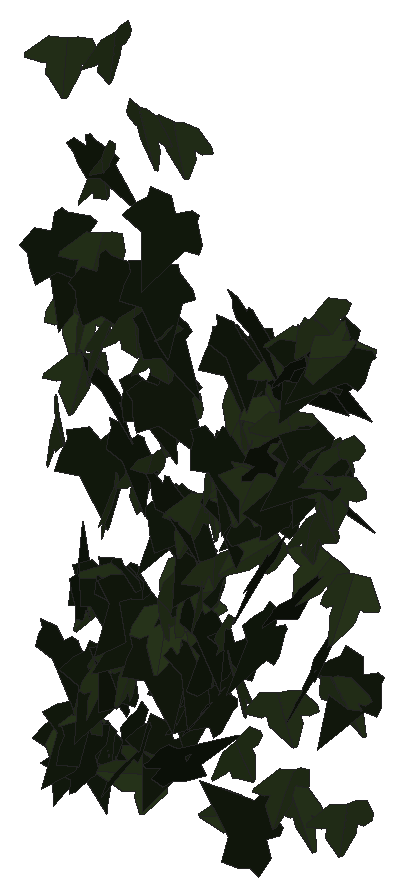
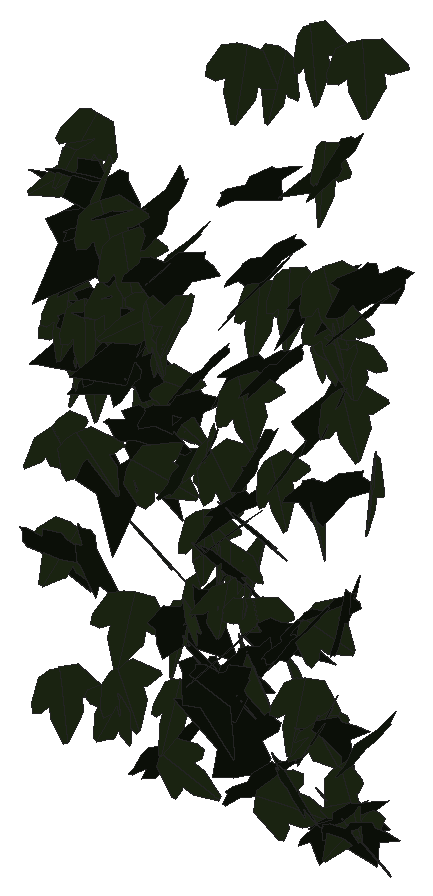
# SketchUp Ruby script. Lengths in inches.
U = 1.inch
M = Sketchup.active_model
def pt(a) = Geom::Point3d.new(a.map { |v| v * U })
def face(e, loops, mat)
  f = e.add_face(loops[0].map { |a| pt(a) })
  loops[1..].each { |l| e.add_face(l.map { |a| pt(a) }).erase! }
  f.material = f.back_material = mat if mat
  f
end
# faces: each face lists its corners as indices into pts; further lists are holes
def faces(e, pts, list, mat = nil) = list.each { |f| face(e, (f[0].is_a?(Array) ? f : [f]).map { |l| l.map { |i| pts[i] } }, mat) }
# xy, xz, yz: faces in a plane at the given z, y or x. An outline is a flat list of corners, or four numbers for a rectangle; further outlines are holes
def ring(l) = l.size == 4 ? [[l[0], l[1]], [l[2], l[1]], [l[2], l[3]], [l[0], l[3]]] : l.each_slice(2).to_a
def flat(e, list, mat, &to3) = list.each { |f| face(e, (f[0].is_a?(Array) ? f : [f]).map { |l| ring(l).map { |u, v| to3.(u, v) } }, mat) }
def xy(e, z, list, mat = nil) = flat(e, list, mat) { |x, y| [x, y, z] }
def xz(e, y, list, mat = nil) = flat(e, list, mat) { |x, z| [x, y, z] }
def yz(e, x, list, mat = nil) = flat(e, list, mat) { |y, z| [x, y, z] }
def lines(e, pts, list) = list.each { |a, b| e.add_line(pt(pts[a]), pt(pts[b])) }
# prism: a flat outline (further loops are holes) pulled along v
def prism(e, loops, v, mat = nil)
  f = face(e, loops, mat); d = Geom::Vector3d.new(v.map { |x| x * U })
  f.pushpull(f.normal.samedirection?(d) ? d.length : -d.length)
end
def box(e, o, s, mat = nil) = prism(e, [[o, [o[0] + s[0], o[1], o[2]], [o[0] + s[0], o[1] + s[1], o[2]], [o[0], o[1] + s[1], o[2]]]], [0, 0, s[2]], mat)
def at(x, y, z, deg = 0) = Geom::Transformation.translation(pt([x, y, z])) * Geom::Transformation.rotation(ORIGIN, Z_AXIS, deg.degrees)
def axes(o, x, y, z) = Geom::Transformation.new([*x, 0, *y, 0, *z, 0, *pt(o).to_a, 1])
def part(name) = M.definitions.add(name)
# library, detail: a bought-in or finely detailed component or shape, given as its bounding box
def library(name, o, s) = part(name).tap { |d| box(d.entities, o, s) }
def detail(e, o, s) = box(e.add_group.entities, o, s)
def put(e, d, t, mat = nil) = e.add_instance(d, t).tap { |i| i.material = mat if mat }
def group(e, t, mat = nil) = e.add_group.tap { |g| g.transformation = t; g.material = mat if mat }.entities
root = M.entities
M.materials.add("efeu1").color = [18, 25, 13]
M.materials.add("efeu2").color = [43, 57, 29]
c1 = part("ivyleaf_10")
p = [[0,0.5,-0.03],[-0.0625,2.02,-0.43],[-0.19,2.01,-0.46],[-0.54,1.05,-0.29],[-0.52,0.625,-0.18],[-0.83,0.76,-0.28],
  [-1.16,0.64,-0.33],[-1.15,0.33,-0.24],[-0.77,-0.39,0.02],[-0.3,-0.51,0.16],[0.04,-0.48,0.23],[-0.02,2.01,-0.4375],
  [-0.06,2.01,-0.43],[0.04,-0.49,0.23],[0.67,-0.49,0.14],[1.38,0.36,-0.2],[1.375,0.51,-0.24],[0.81,0.65,-0.19],
  [0.62,0.59,-0.15],[0.6,1.09,-0.28],[0.5,1.23,-0.31]]
faces(c1.entities,p,[[0,1,2,3,4,5,6,7,8,9,10],[11,12,0,13,14,15,16,17,18,19,20]],"efeu2")
c2 = part("ivyleaf_9")
p = [[1.54,2.16,1.25],[1.36,2.04,1.19],[-0.21,0.99,0.68],[-0.71,1.11,0.82],[-0.85,0.86,0.67],[-0.8,0.17,0.21],
  [-0.9,-0.01,0.1],[-0.67,-0.16,-0.02],[-0.08,-0.08,-0.05],[-0.03,-0.6,-0.4],[0.65,-0.88,-0.66],[0.83,-0.6,-0.49],
  [1.29,-0.42,-0.43],[1.8125,-0.07,-0.26],[1.21,0.44,0.15]]
faces(c2.entities,p,[[0,1,2,3,4,5,6,7,8,9,10,11,12,13,14]],"efeu1")
put(root,c1,axes([562.84,127.59,257.41],[0.41303,-0.76351,-0.7131],[-0.09509,0.73616,-0.84327],[1.0404,0.37039,0.20603]))
put(root,c2,axes([562.25,128.91,247.09],[0.18031,-0.95699,0.36294],[0.20425,-0.32748,-0.96494],[1.00292,0.23875,0.13126]))
put(root,c2,axes([562.58,127.88,265.38],[0.22614,-0.63801,-0.89851],[0.05984,0.92299,-0.64034],[1.10036,0.08093,0.21948]))
put(root,c2,axes([563.07,128.88,243.53],[-0.73357,-0.65535,-0.20186],[0.21145,0.06502,-0.9795],[0.65232,-0.75806,0.09049]))
put(root,c1,axes([563.75,128.37,244.99],[-0.7587,0.15917,0.7499],[-0.74689,0.08426,-0.77354],[-0.17274,-1.06342,0.05095]))
put(root,c2,axes([562.89,128.7,263.84],[-0.16436,-1.00943,0.40946],[0.11007,-0.42737,-1.00939],[1.08374,-0.10968,0.16461]))
put(root,c1,axes([563.41,127.64,273.79],[-0.83592,-0.75041,0.11104],[-0.01136,-0.15283,-1.11835],[0.75849,-0.8293,0.10562]))
put(root,c2,axes([563.48,129.04,243.86],[-0.63138,-0.80957,0.35535],[-0.14365,-0.33692,-1.02282],[0.87238,-0.6414,0.08876]))
put(root,c1,axes([563.04,128.13,243.67],[0.40834,0.68659,0.64921],[0.32372,0.56279,-0.79881],[-0.88774,0.52104,0.00733]))
put(root,c1,axes([563.73,128.17,259.99],[-0.44641,-0.98521,0.21774],[-0.00764,-0.2348,-1.07802],[1.00895,-0.43768,0.08817]))
put(root,c1,axes([563.39,128.36,262.37],[1.04935,0.34469,0.06041],[0.06179,0.00547,-1.10443],[-0.34445,1.05108,-0.01407]))
put(root,c1,axes([563.98,128.51,263.49],[-1.02158,-0.29347,0.28723],[-0.25696,-0.14386,-1.06091],[0.32031,-1.0514,0.06499]))
put(root,c2,axes([564.42,127.89,243.42],[-0.78664,0.6294,0.42305],[-0.35232,0.23647,-1.00692],[-0.67156,-0.86131,0.03271]))
put(root,c1,axes([564.05,128.8,265.03],[-0.49407,-0.95007,0.25956],[0.00953,-0.29498,-1.06161],[0.98484,-0.47378,0.14048]))
put(root,c2,axes([563.69,128.74,243.64],[0.0197,-0.96646,-0.33025],[0.01052,0.33048,-0.96652],[1.02127,0.01524,0.01633]))
put(root,c1,axes([564,128.18,263.08],[0.45011,-0.89395,0.51532],[0.33214,-0.40677,-0.99575],[0.97693,0.55017,0.10111]))
put(root,c2,axes([564.57,127.26,250.3125],[-0.0748,-0.53798,0.91294],[0.12584,0.90423,0.54316],[-1.05217,0.14639,0.00006]))
put(root,c2,axes([564.67,128.71,246.86],[-0.74485,-0.7469,-0.04319],[0.03003,0.03105,-1.05483],[0.74755,-0.74545,-0.00066]))
put(root,c1,axes([564.72,128.43,246.74],[0.35635,0.86532,-0.42603],[-0.24336,-0.35882,-0.93236],[-0.93331,0.42396,0.08045]))
put(root,c2,axes([564.39,128.41,256.67],[-0.29435,-0.98666,-0.40915],[0.18504,0.37088,-1.0275],[1.05198,-0.34131,0.06625]))
put(root,c1,axes([564.9,128.42,250.83],[-0.19144,-0.69625,0.81307],[-0.02881,-0.82232,-0.71096],[1.07006,-0.1467,0.12632]))
put(root,c2,axes([564.09,128.12,269.44],[0.77749,-0.80115,-0.05837],[0.1467,0.22148,-1.08589],[0.78976,0.74756,0.25917]))
put(root,c1,axes([564.91,128.51,274.27],[-0.05622,-1.10216,-0.15484],[-0.00472,0.15527,-1.10352],[1.11298,-0.05501,-0.01251]))
put(root,c1,axes([564.93,127.75,269.21],[0.11433,-1.03129,-0.49062],[0.0073,0.49372,-1.03611],[1.14202,0.10009,0.05574]))
put(root,c2,axes([564.17,128.61,259.58],[0.61067,-0.84668,0.39602],[0.22897,-0.32313,-1.04392],[0.90624,0.65218,-0.0031]))
put(root,c1,axes([565,127.94,261.96],[0.34847,-0.95776,0.37295],[0.11955,-0.35336,-1.01915],[1.02084,0.36832,-0.00796]))
put(root,c2,axes([564.68,128.91,246.48],[-0.05787,-0.59802,0.85251],[0.09056,-0.85348,-0.59256],[1.03741,0.04114,0.09928]))
put(root,c1,axes([565.16,128.76,248.15],[-0.489,-0.9112,-0.30006],[0.14835,0.26092,-1.03409],[0.94779,-0.51096,0.00704]))
put(root,c2,axes([564.81,128.1,251.3],[0.01367,-0.99533,-0.36117],[0.03973,0.36142,-0.99454],[1.05809,-0.00071,0.04201]))
put(root,c2,axes([564.77,127.86,264.34],[0.43933,-0.82855,-0.72022],[-0.14699,0.72437,-0.92299],[1.08794,0.43246,0.16613]))
put(root,c2,axes([564.9,129.16,250.83],[0.26115,-1.06639,0.03219],[0.00673,-0.03149,-1.0979],[1.06685,0.26123,-0.00095]))
put(root,c1,axes([565.55,127.65,255.29],[0.51777,-0.93369,-0.10677],[-0.0372,0.10144,-1.06751],[0.93904,0.51884,0.01658]))
put(root,c2,axes([565.98,128.86,244.72],[-0.89666,0.26347,-0.4856],[0.43999,-0.21931,-0.93142],[-0.33413,-0.99585,0.07665]))
put(root,c2,axes([565.85,128.93,250.14],[-0.37368,-0.83565,0.61182],[-0.18038,-0.58797,-0.91325],[1.01985,-0.41018,0.06266]))
put(root,c1,axes([566.82,128.34,243.22],[0.20289,0.05653,-1.1268],[-1.12804,-0.01,-0.20361],[-0.01987,1.14487,0.05386]))
put(root,c2,axes([565.77,128.57,257.15],[0.30939,-0.98509,0.32567],[0.12484,-0.30203,-1.03217],[1.02999,0.33251,0.02728]))
put(root,c1,axes([566.41,127.71,248.21],[0.80744,-0.71475,-0.19769],[-0.14626,0.13303,-1.07835],[0.72702,0.82058,0.00262]))
put(root,c1,axes([566.5625,128.5625,256.44],[-0.05873,-1.07905,0.08087],[0.01241,-0.08166,-1.08052],[1.08201,-0.05764,0.01678]))
put(root,c1,axes([566.74,127.48,263.41],[-0.17401,-1.07449,-0.26448],[0.06053,0.25809,-1.08834],[1.1049,-0.18336,0.01797]))
put(root,c2,axes([567.14,128.35,249.73],[-0.90558,-0.38315,0.30559],[-0.27275,-0.13943,-0.98307],[0.40718,-0.94552,0.02113]))
put(root,c1,axes([567.17,127.59,272.1],[-1.07615,0.34445,-0.02824],[0.01274,-0.05275,-1.12898],[-0.34537,-1.07522,0.04634]))
put(root,c2,axes([567.04,129.37,244.28],[-0.36091,-0.94212,0.23799],[-0.04425,-0.23767,-1.00799],[0.9707,-0.36112,0.04253]))
put(root,c1,axes([566.78,129.05,247.7],[0.62974,-0.51065,-0.74179],[0.57998,-0.46249,0.81075],[-0.68894,-0.85611,0.00447]))
put(root,c2,axes([566.98,128.01,260.3],[0.32554,-0.96621,-0.38496],[-0.07583,0.38025,-1.01852],[1.0373,0.33102,0.04636]))
put(root,c2,axes([567.68,129.26,254.57],[-0.98097,-0.11127,-0.32265],[0.33868,-0.19605,-0.96211],[0.04217,-1.01389,0.22145]))
put(root,c2,axes([567.16,128.48,264.81],[-0.00108,-1.09219,-0.16823],[0.03923,0.16809,-1.0915],[1.10437,-0.00704,0.03861]))
put(root,c1,axes([567.83,128.82,259.32],[-0.41631,-1.00282,0.18365],[0.00524,-0.20047,-1.08281],[1.01949,-0.40847,0.08055]))
put(root,c2,axes([567.74,128.63,267.59],[-0.48232,-0.98023,0.18834],[0.01651,-0.21698,-1.08702],[0.99803,-0.47013,0.109]))
put(root,c2,axes([567.52,128.23,248.9375],[-0.10611,-1.01434,-0.32948],[0.06465,0.32438,-1.01946],[1.06455,-0.1208,0.02907]))
put(root,c1,axes([567.78,128.11,250.4],[0.9029,0.57529,-0.10566],[-0.09884,-0.04148,-1.07045],[-0.5765,0.90811,0.01804]))
put(root,c1,axes([567.97,127.65,262.57],[-0.1996,-1.03459,-0.33106],[0.08726,0.32024,-1.0534],[1.08276,-0.21653,0.02387]))
put(root,c2,axes([567.56,128.05,260.32],[0.25415,-0.85668,-0.61589],[0.15235,0.65666,-0.85053],[1.04404,0.11272,0.27404]))
put(root,c1,axes([568.49,127.16,251.72],[-0.29318,0.64958,0.78832],[-0.48687,0.63213,-0.70194],[-0.89797,-0.55481,0.12321]))
put(root,c2,axes([567.71,127.81,263.32],[0.54242,-0.93965,-0.3083],[-0.0252,0.33838,-1.07568],[0.98861,0.52419,0.14173]))
put(root,c2,axes([567.8125,128.57,255.07],[0.38522,-0.85605,-0.58965],[0.06219,0.64669,-0.89823],[1.03761,0.27906,0.27275]))
put(root,c1,axes([568.5625,127.88,271.89],[-1.12362,-0.12835,0.03775],[-0.03844,0.00396,-1.1309],[0.12815,-1.12425,-0.00829]))
put(root,c2,axes([567.85,127.97,256.16],[0.65181,-0.8578,0.06357],[0.03328,-0.05455,-1.07733],[0.85951,0.65263,-0.0065]))
put(root,c2,axes([569.06,129.13,252.56],[-1.04243,-0.01938,-0.09874],[0.10025,-0.11215,-1.03642],[0.00861,-1.04107,0.11349]))
put(root,c2,axes([568.64,128.9375,247.82],[-0.68242,-0.72357,-0.43124],[0.29453,0.315,-0.99461],[0.78916,-0.74326,-0.0017]))
put(root,c1,axes([568.49,128.48,252.57],[1.0637,-0.08077,0.312],[0.31023,-0.03493,-1.06671],[0.08732,1.10796,-0.01088]))
put(root,c1,axes([568.72,128.63,250.98],[0.18588,1.01356,0.0054],[0.00079,0.00535,-1.03046],[-1.01358,0.18588,0.00019]))
put(root,c2,axes([568.72,129.14,253.11],[-0.33325,-0.84696,0.56115],[0.07978,-0.61055,-0.87415],[1.01285,-0.23057,0.25348]))
put(root,c2,axes([568.38,127.26,244.57],[0.48141,0.90677,-0.46551],[0.18378,0.42916,1.02603],[1.00257,-0.51408,0.03545]))
put(root,c1,axes([569.25,128.35,255.74],[-0.19973,-1.01756,0.40443],[-0.00609,-0.41007,-1.03475],[1.09497,-0.18789,0.06801]))
put(root,c2,axes([568.79,129.17,248.34],[-0.1413,-0.97988,0.5077],[0.11633,-0.52221,-0.97552],[1.09745,-0.07081,0.16877]))
put(root,c2,axes([569.71,128.52,247.3],[-0.42437,0.97747,-0.16961],[0.05207,-0.16227,-1.06549],[-0.99071,-0.42723,0.01665]))
put(root,c1,axes([569.47,128.02,252.23],[0.47023,-0.78912,-0.53773],[-0.12007,0.54577,-0.90592],[0.94733,0.46087,0.15209]))
put(root,c1,axes([569.53,128.77,256.54],[-0.2213,0.99873,-0.22509],[0.01098,-0.22796,-1.02226],[-1.02373,-0.21834,0.03769]))
put(root,c1,axes([569.74,128.53,253.21],[-0.32208,-0.98323,-0.10761],[0.07323,0.08916,-1.03381],[0.98639,-0.32767,0.04161]))
put(root,c2,axes([570.41,128.41,247.99],[-1.06753,0.36853,0.09714],[-0.0941,0.02508,-1.12933],[-0.36932,-1.07165,0.00698]))
put(root,c2,axes([569.3,128.6,250.8],[0.31849,-1.00713,0.35708],[0.15149,-0.32628,-1.05539],[1.05777,0.34997,0.04363]))
put(root,c2,axes([570.35,128.92,249.8125],[0.01598,0.38777,-0.98513],[0.02707,-0.98507,-0.38731],[-1.05836,-0.01934,-0.02478]))
put(root,c1,axes([569.9375,129.09,250.23],[0.4319,-0.72874,0.63942],[0.35789,-0.53071,-0.84659],[0.90102,0.56012,0.02976]))
put(root,c1,axes([571.28,128.28,243.11],[0.41562,0.00843,-0.96101],[-0.93681,0.2372,-0.40308],[0.21446,1.01981,0.1017]))
put(root,c2,axes([570.08,129.13,255.43],[0.10528,-0.89986,0.58289],[0.29415,-0.53898,-0.8852],[1.03102,0.24566,0.19303]))
put(root,c2,axes([570.6,129.28,257.98],[-0.50856,-0.94321,-0.09432],[0.03011,0.0909,-1.07145],[0.94743,-0.50918,-0.01657]))
put(root,c2,axes([570.29,128.05,258.98],[0.31241,-1.02655,-0.16373],[-0.02957,0.16212,-1.07287],[1.03911,0.31325,0.0187]))
put(root,c1,axes([570.9,128.43,249.05],[-0.85525,0.5965,0.21832],[-0.18585,0.11515,-1.04266],[-0.6074,-0.87514,0.01161]))
put(root,c1,axes([571.66,128.45,257.375],[0.58484,-0.02398,-0.89333],[-0.88158,0.15942,-0.58143],[0.1464,1.05578,0.06751]))
put(root,c1,axes([571.08,128.36,245.88],[-0.19469,-0.93343,-0.45534],[0.16592,0.42937,-0.95112],[1.02523,-0.24674,0.06745]))
put(root,c1,axes([571.2,128.1,261.2],[-0.08866,0.98331,0.40809],[-0.06157,0.40408,-0.98703],[-1.06284,-0.10544,0.02314]))
put(root,c2,axes([571.21,128.8,263.25],[-0.44044,-0.94982,-0.47901],[0.18961,0.44005,-1.0469],[1.04673,-0.47937,-0.01192]))
put(root,c1,axes([572.08,128.89,254.81],[-0.35438,-0.45566,0.90524],[-0.47919,-0.76968,-0.57501],[0.89301,-0.59383,0.05068]))
put(root,c2,axes([571.1,128.5625,263.41],[0.111,-1.03991,0.36563],[0.19459,-0.34322,-1.03525],[1.085,0.16794,0.14827]))
put(root,c1,axes([571.74,128.95,261.03],[0.33805,-1.0447,-0.00092],[0.00655,0.00309,-1.09801],[1.04468,0.33804,0.00718]))
put(root,c1,axes([572.03,128.1,257.85],[-0.74531,-0.64198,0.39704],[-0.22776,-0.3407,-0.97842],[0.71965,-0.77269,0.10154]))
put(root,c1,axes([571.68,128.25,260.41],[-0.27223,1.02654,0.03381],[-0.02357,0.02873,-1.06191],[-1.02683,-0.27281,0.01542]))
put(root,c2,axes([572.4,128.17,242.54],[-0.31186,-1.12062,-0.0585],[0.02162,-0.0667,1.16257],[-1.12194,0.31021,0.03866]))
put(root,c2,axes([572.375,129.41,256.84],[-0.94417,-0.47383,0.23394],[-0.22005,-0.08294,-1.05612],[0.48044,-0.96918,-0.02399]))
put(root,c2,axes([571.6875,128.1875,264.93],[0.57803,-0.85402,0.42106],[0.22345,-0.35716,-1.03115],[0.92559,0.61956,-0.01401]))
put(root,c2,axes([572.83,128.23,251.6875],[-0.97341,0.08254,-0.36864],[0.34915,-0.19245,-0.96503],[-0.14423,-1.02293,0.15181]))
put(root,c1,axes([572.19,127.9375,260.6],[-0.29594,-0.37462,-1.03871],[0.85424,0.60372,-0.46113],[0.69967,-0.89556,0.12365]))
put(root,c2,axes([573.02,127.72,254.98],[-0.57962,0.75082,-0.54968],[0.36024,-0.41604,-0.94814],[-0.85797,-0.68192,-0.02675]))
put(root,c2,axes([573.7,128.03,257.4375],[-0.74662,0.60353,0.50151],[-0.49845,0.16988,-0.94652],[-0.60606,-0.88323,0.16064]))
put(root,c2,axes([572.45,127.87,258.82],[0.55423,0.4218,0.90625],[0.67719,0.60377,-0.69516],[-0.73526,0.87403,0.04286]))
put(root,c1,axes([573.14,128.72,263.17],[-0.41742,-1.01685,0.1269],[0.02661,-0.14773,-1.09627],[1.0244,-0.41051,0.08019]))
put(root,c1,axes([573.18,128.36,248.62],[-0.92946,-0.55922,-0.16061],[0.14615,0.06859,-1.0846],[0.56317,-0.94074,0.01639]))
put(root,c1,axes([573.68,128.22,260.93],[-0.88787,-0.6538,0.00865],[0.00258,-0.0181,-1.1025],[0.65385,-0.88773,0.0161]))
put(root,c1,axes([573.66,128.22,245.47],[-0.29365,-0.9536,0.29057],[-0.00272,-0.30214,-0.99434],[0.99688,-0.28172,0.08287]))
put(root,c2,axes([572.93,128.64,258.68],[0.9549,-0.45932,0.18687],[0.19317,-0.02888,-1.0581],[0.45671,0.97258,0.05683]))
put(root,c1,axes([573.88,128.98,264.31],[-0.60027,-0.87702,0.25844],[-0.05892,-0.27142,-1.0579],[0.91241,-0.59452,0.10172]))
put(root,c2,axes([574.13,127.8125,253.63],[0.03511,1.09872,0.11527],[-0.00339,0.11544,-1.09926],[-1.10474,0.03457,0.00704]))
put(root,c1,axes([574.31,128.08,259.6],[-0.92636,-0.28371,0.44612],[-0.40102,-0.20944,-0.96591],[0.34453,-1.00663,0.07523]))
put(root,c1,axes([573.81,128.51,244.55],[-0.88451,0.17651,-0.46194],[0.39206,-0.32662,-0.8755],[-0.30139,-0.9429,0.2168]))
put(root,c1,axes([574.76,129.01,254.79],[-0.79732,-0.32726,0.62113],[-0.45133,-0.48102,-0.83279],[0.53778,-0.8889,0.22198]))
put(root,c2,axes([574.59,129.18,250.88],[-0.74218,0.35638,-0.65274],[0.52903,-0.39515,-0.81725],[-0.52269,-0.90596,0.09968]))
put(root,c2,axes([574.46,128.96,263.77],[-0.59529,-0.88266,0.24229],[0.02913,-0.30715,-1.04736],[0.91485,-0.56456,0.191]))
put(root,c2,axes([574.32,127.63,263.18],[0.89833,0.62592,0.15329],[0.13499,0.07438,-1.09477],[-0.63012,0.90827,-0.01599]))
put(root,c2,axes([575.07,127.33,264.56],[0.05255,1.09647,0.03541],[0.00258,0.03532,-1.09773],[-1.09704,0.0526,-0.00089]))
put(root,c1,axes([574.83,127.76,265.1],[-0.52506,0.94034,0.09055],[-0.02829,0.0879,-1.07685],[-0.94426,-0.52551,-0.01808]))
put(root,c1,axes([575,128.6,259.8125],[-0.28283,-1.02643,-0.11188],[0.05404,0.10113,-1.06438],[1.03109,-0.28685,0.02509]))
put(root,c2,axes([574.92,128.7,259.96],[-0.57617,-0.91367,0.00551],[0.00076,-0.007,-1.08016],[0.91369,-0.57615,0.00438]))
put(root,c2,axes([575.41,128.26,260.03],[-0.96454,-0.43895,0.26583],[-0.23066,-0.13473,-1.0594],[0.45841,-0.99139,0.02627]))
put(root,c2,axes([574.56,128.39,262.9375],[1.00746,0.44244,0.15073],[0.1413,0.05309,-1.1003],[-0.44554,1.01729,-0.00813]))
put(root,c1,axes([575.375,127.75,257.53],[-0.01581,-1.0904,-0.1279],[0.01313,0.12772,-1.09045],[1.09779,-0.01723,0.0112]))
put(root,c2,axes([574.58,128.28,258.77],[0.9681,-0.29411,0.40294],[0.37897,-0.13848,-1.01158],[0.32442,1.03943,-0.02076]))
put(root,c1,axes([575.69,127.58,257.95],[0.19281,-0.88227,-0.62108],[0.12123,0.64464,-0.8781],[1.07212,0.08578,0.21099]))
put(root,c1,axes([575.78,128.53,260.15],[-0.31542,-1.02853,-0.2291],[0.18481,0.18144,-1.069],[1.0374,-0.34504,0.12078]))
put(root,c1,axes([576.04,127.91,259.16],[-0.85397,-0.65551,0.03164],[-0.02451,-0.02003,-1.07656],[0.65582,-0.85433,0.00096]))
put(root,c1,axes([576.06,128.625,244.72],[-0.54954,-0.90199,0.0654],[-0.03173,-0.05725,-1.05621],[0.9038,-0.55045,0.00268]))
put(root,c1,axes([575.82,127.33,266.42],[-0.32881,-0.84895,-0.72925],[0.38321,0.62872,-0.90471],[1.05151,-0.4946,0.10167]))
put(root,c2,axes([576.45,128.52,264.94],[-1.02467,-0.36465,0.15589],[-0.03739,-0.34117,-1.04376],[0.39481,-0.97871,0.30576]))
put(root,c1,axes([576.05,128.25,250.29],[-0.9818,0.10934,-0.37482],[0.37221,-0.04422,-0.98787],[-0.11792,-1.04999,0.00257]))
put(root,c2,axes([576.47,129.03,250.55],[-1.02141,-0.32738,-0.21895],[0.21493,0.04662,-1.07239],[0.33003,-1.04357,0.02078]))
put(root,c1,axes([575.94,127.34,264.99],[-0.07092,-0.29719,-1.1275],[0.63091,0.94017,-0.2875],[0.98058,-0.6264,0.10343]))
put(root,c1,axes([576.36,128.54,254.55],[0.36374,0.91566,-0.48714],[-0.23214,-0.43126,-0.98395],[-1.01086,0.42851,0.05067]))
